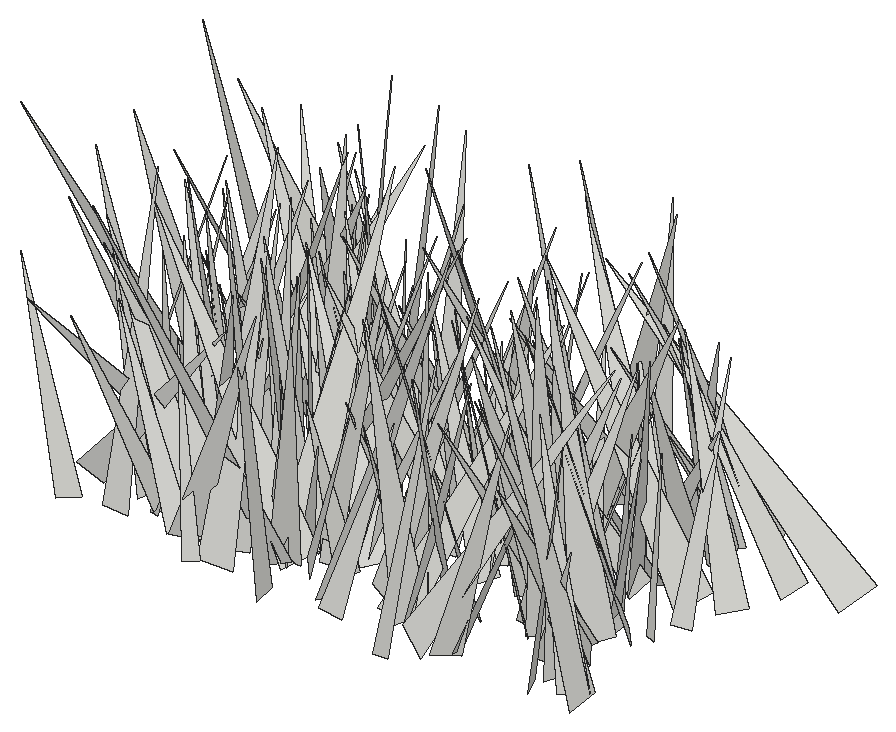
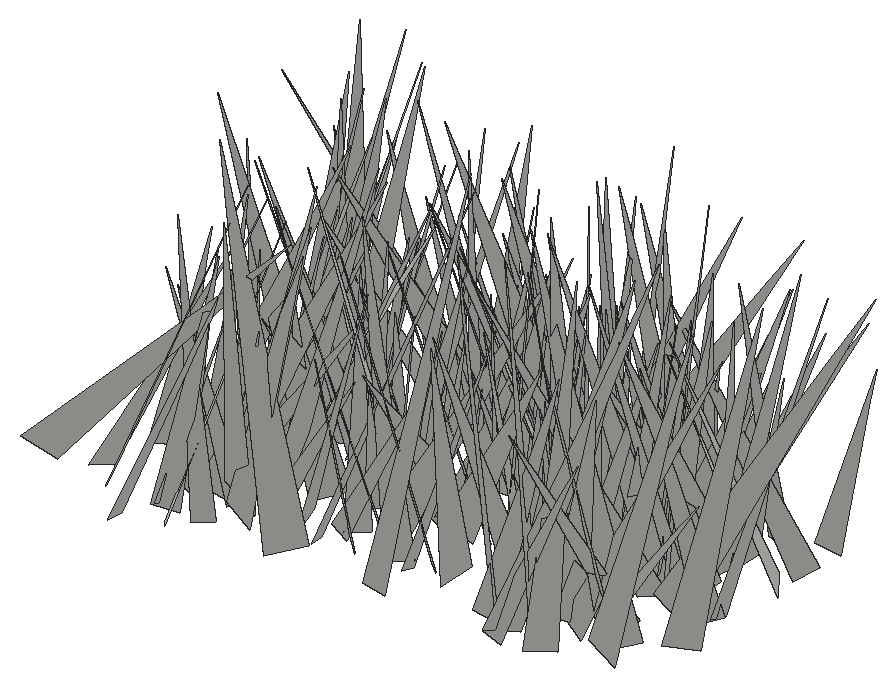
# SketchUp Ruby script. Lengths in inches.
U = 1.inch
M = Sketchup.active_model
def pt(a) = Geom::Point3d.new(a.map { |v| v * U })
def face(e, loops, mat)
  f = e.add_face(loops[0].map { |a| pt(a) })
  loops[1..].each { |l| e.add_face(l.map { |a| pt(a) }).erase! }
  f.material = f.back_material = mat if mat
  f
end
# faces: each face lists its corners as indices into pts; further lists are holes
def faces(e, pts, list, mat = nil) = list.each { |f| face(e, (f[0].is_a?(Array) ? f : [f]).map { |l| l.map { |i| pts[i] } }, mat) }
# xy, xz, yz: faces in a plane at the given z, y or x. An outline is a flat list of corners, or four numbers for a rectangle; further outlines are holes
def ring(l) = l.size == 4 ? [[l[0], l[1]], [l[2], l[1]], [l[2], l[3]], [l[0], l[3]]] : l.each_slice(2).to_a
def flat(e, list, mat, &to3) = list.each { |f| face(e, (f[0].is_a?(Array) ? f : [f]).map { |l| ring(l).map { |u, v| to3.(u, v) } }, mat) }
def xy(e, z, list, mat = nil) = flat(e, list, mat) { |x, y| [x, y, z] }
def xz(e, y, list, mat = nil) = flat(e, list, mat) { |x, z| [x, y, z] }
def yz(e, x, list, mat = nil) = flat(e, list, mat) { |y, z| [x, y, z] }
def lines(e, pts, list) = list.each { |a, b| e.add_line(pt(pts[a]), pt(pts[b])) }
# prism: a flat outline (further loops are holes) pulled along v
def prism(e, loops, v, mat = nil)
  f = face(e, loops, mat); d = Geom::Vector3d.new(v.map { |x| x * U })
  f.pushpull(f.normal.samedirection?(d) ? d.length : -d.length)
end
def box(e, o, s, mat = nil) = prism(e, [[o, [o[0] + s[0], o[1], o[2]], [o[0] + s[0], o[1] + s[1], o[2]], [o[0], o[1] + s[1], o[2]]]], [0, 0, s[2]], mat)
def at(x, y, z, deg = 0) = Geom::Transformation.translation(pt([x, y, z])) * Geom::Transformation.rotation(ORIGIN, Z_AXIS, deg.degrees)
def axes(o, x, y, z) = Geom::Transformation.new([*x, 0, *y, 0, *z, 0, *pt(o).to_a, 1])
def part(name) = M.definitions.add(name)
# library, detail: a bought-in or finely detailed component or shape, given as its bounding box
def library(name, o, s) = part(name).tap { |d| box(d.entities, o, s) }
def detail(e, o, s) = box(e.add_group.entities, o, s)
def put(e, d, t, mat = nil) = e.add_instance(d, t).tap { |i| i.material = mat if mat }
def group(e, t, mat = nil) = e.add_group.tap { |g| g.transformation = t; g.material = mat if mat }.entities
root = M.entities
c1 = part("fur_instance\#9")
p = [[0.8125,0,1.79],[0.67,-0.02,1.48],[0,-0.11,0],[0,0.11,0]]
faces(c1.entities,p,[[0,1,2,3]])
put(root,c1,axes([480.03,113.66,-21.86],[-7.83982,-0.95667,1.33619],[-0.96404,7.9519,0.03699],[1.33088,0.12461,7.89789]))
put(root,c1,axes([473.71,113.29,-21.86],[4.65487,-3.05281,1.35089],[-3.29302,-4.57961,0.99778],[-0.54826,1.58741,5.47649]))
put(root,c1,axes([465.41,112.65,-21.86],[-7.60319,-2.30719,2.08818],[-2.71089,7.61771,-1.45385],[1.52798,2.03457,7.8114]))
put(root,c1,axes([468.28,113.08,-21.86],[-0.49271,4.25835,1.65602],[4.30491,0.99075,-1.26683],[1.53091,-1.41548,4.0953]))
put(root,c1,axes([460.34,114.23,-21.86],[3.9818,-4.86666,0.84742],[-4.90357,-3.76221,1.43455],[0.59785,1.55519,6.12218]))
put(root,c1,axes([477.73,113.43,-21.86],[4.582,2.26461,1.64468],[2.3704,-4.81752,0.02956],[-1.48816,-0.70087,5.111]))
put(root,c1,axes([470.9,114.64,-21.86],[-5.74569,2.33772,2.68731],[2.89131,6.03979,0.92776],[2.08013,-1.9379,6.13328]))
put(root,c1,axes([464.3125,115.25,-21.86],[1.6892,-5.96403,1.00433],[-6.01842,-1.55459,0.89085],[0.59746,1.20222,6.13428]))
put(root,c1,axes([458.59,115.15,-21.66],[0.69444,-4.60057,1.02449],[-4.36557,-1.0182,-1.61314],[-1.77671,0.70364,4.36409]))
put(root,c1,axes([472.04,111.39,-21.66],[2.45384,5.3856,0.3895],[5.06414,-2.44383,1.88676],[-1.87372,0.44803,5.60947]))
put(root,c1,axes([478,116.68,-21.66],[-5.39374,-4.42373,0.73063],[-4.15874,5.36317,1.77113],[1.67573,-0.92879,6.74722]))
put(root,c1,axes([465.64,115.03,-21.66],[3.73133,2.74864,1.27928],[3.02044,-3.19509,-1.94493],[0.26177,-2.31318,4.20655]))
put(root,c1,axes([455.11,113.64,-21.66],[-1.60239,4.56784,1.22355],[4.62571,1.24567,1.40748],[-0.98238,-1.58525,4.63161]))
put(root,c1,axes([477.46,116.94,-21.86],[4.02503,-3.95124,0.17731],[-3.62061,-3.78264,-2.10414],[-1.59215,-1.38705,5.23314]))
put(root,c1,axes([469.98,115.76,-21.86],[-3.99319,-2.60087,1.40659],[-2.16034,4.18012,1.59628],[2.0189,-0.6713,4.49021]))
put(root,c1,axes([479.35,113.98,-21.86],[1.60632,-4.77246,2.92285],[-5.28453,-2.29441,-0.84211],[-1.84207,2.42054,4.96463]))
put(root,c1,axes([461.57,112.97,-21.86],[-0.27528,4.26527,0.41219],[4.05575,0.12601,1.40472],[-1.38323,-0.47937,4.03672]))
put(root,c1,axes([464.38,114.92,-21.86],[-3.051,-7.21191,1.32168],[-6.61753,2.09219,-3.8598],[-3.15701,2.58422,6.81338]))
put(root,c1,axes([471.67,116.11,-21.86],[-2.94569,-5.43055,1.36405],[-5.282,3.20651,1.35919],[1.85796,0.50597,6.02666]))
put(root,c1,axes([476.96,115.25,-21.86],[1.46313,-3.34357,0.17988],[-3.25058,-1.37123,0.95187],[0.80348,0.54115,3.52337]))
put(root,c1,axes([472.27,113.01,-21.66],[3.56611,7.00423,0.23479],[6.50816,-3.2121,-3.02618],[2.59966,-1.56674,7.25387]))
put(root,c1,axes([460,114.21,-21.66],[-2.19401,4.08598,0.64459],[3.98986,1.89782,1.55038],[-1.09165,-1.27572,4.37096]))
put(root,c1,axes([466.98,115.75,-21.86],[3.15907,-2.58161,1.45094],[-2.40771,-3.47422,-0.93937],[-1.72421,0.12146,3.97014]))
put(root,c1,axes([463.96,115.18,-21.86],[2.13967,5.72529,2.72362],[6.33838,-1.99885,-0.77766],[-0.14822,-2.82858,6.06237]))
put(root,c1,axes([464.82,115.5625,-21.86],[-6.95314,3.37085,0.59923],[3.40426,6.66259,2.02209],[-0.36434,-2.07731,7.45788]))
put(root,c1,axes([464.26,116.6875,-21.86],[-0.71595,-3.844,0.50308],[-3.36107,0.87042,1.86752],[1.93201,0.08975,3.4353]))
put(root,c1,axes([460.83,114.49,-21.86],[3.00603,-4.02582,3.59921],[-4.80148,-3.87769,-0.32715],[-2.47129,2.63706,5.01362]))
put(root,c1,axes([454.53,115.67,-21.66],[2.58062,-5.27777,0.62862],[-4.46822,-1.77579,3.43383],[2.87837,1.97518,4.76689]))
put(root,c1,axes([459.5,117.1,-21.66],[6.23542,-1.61716,0.46655],[-1.48447,-6.12774,-1.40019],[-0.79324,-1.24458,6.2877]))
put(root,c1,axes([475.46,117.84,-21.66],[5.45366,-4.66647,1.60556],[-4.21255,-5.64853,-2.10822],[-2.57063,-0.64365,6.86103]))
put(root,c1,axes([459.94,115.625,-21.66],[-5.34119,3.3335,0.99515],[3.47843,5.14626,1.43085],[0.05516,-1.74201,6.13133]))
put(root,c1,axes([469.27,115.0625,-21.66],[2.86437,6.58912,2.04567],[6.83224,-2.40073,-1.83379],[0.96006,-2.57407,6.94682]))
put(root,c1,axes([470.81,114.93,-21.86],[5.20805,0.62891,1.21236],[0.54515,-5.33937,0.42794],[-1.25226,0.29119,5.2284]))
put(root,c1,axes([457.89,119.08,-21.86],[3.04305,-5.48081,0.27728],[-4.42438,-2.6378,-3.58374],[-3.24669,-1.54241,5.14356]))
put(root,c1,axes([467.7,113.82,-21.66],[7.57177,-0.43303,1.80554],[-0.88332,-7.50835,1.90355],[-1.63317,2.05334,7.34137]))
put(root,c1,axes([472.63,116.49,-21.86],[-4.6315,-5.30606,1.24554],[-5.44783,4.55599,-0.84886],[0.16366,1.49838,6.99175]))
put(root,c1,axes([475.89,116.82,-21.86],[3.80262,-6.94068,2.14426],[-7.19034,-3.9408,-0.00453],[-1.0344,1.87826,7.9141]))
put(root,c1,axes([462.51,113.27,-21.86],[0.64716,8.27924,1.09317],[8.31403,-0.74193,0.69715],[-0.78591,-1.0312,8.27518]))
put(root,c1,axes([463.42,116.51,-21.86],[2.3019,2.88607,2.09295],[3.52279,-2.224,-0.8077],[-0.54756,-2.17555,3.60219]))
put(root,c1,axes([456.9,114.2,-21.86],[1.29784,6.7007,1.25957],[6.74597,-1.44798,0.75208],[-0.98888,-1.08363,6.78367]))
put(root,c1,axes([473.94,119.3125,-21.86],[-4.9139,-3.74374,0.55427],[-3.15126,4.55055,2.79845],[2.0958,-1.9355,5.50733]))
put(root,c1,axes([459.28,117.84,-21.66],[3.15853,-4.87453,2.05329],[-4.28659,-3.76007,-2.33247],[-3.09874,0.23284,5.31949]))
put(root,c1,axes([470.83,115.28,-21.86],[2.86323,5.98862,2.41998],[6.20716,-3.28322,0.78076],[-1.78634,-1.80966,6.59182]))
put(root,c1,axes([478.1,114.54,-21.86],[-7.47088,0.3057,1.86762],[-0.12287,7.51123,-1.721],[1.88848,1.69808,7.27638]))
put(root,c1,axes([474.64,117.06,-21.86],[0.98375,-3.96673,0.69714],[-3.91068,-0.76919,1.14174],[0.96305,0.9285,3.92417]))
put(root,c1,axes([469.9,115.8,-21.86],[-5.58164,-0.15602,0.84627],[-0.25003,5.60842,-0.61509],[0.82341,0.64537,5.54984]))
put(root,c1,axes([462.73,117.91,-21.86],[-2.8459,-6.01928,1.64103],[-5.98512,3.14324,1.14988],[1.76154,0.95508,6.5581]))
put(root,c1,axes([465.44,116.35,-21.86],[2.35807,6.09522,2.44102],[6.53945,-1.94795,-1.45322],[0.58808,-2.77931,6.37184]))
put(root,c1,axes([473.87,113.78,-21.86],[5.28462,2.45266,0.54887],[2.09175,-5.00051,2.20534],[-1.39334,1.79538,5.39252]))
put(root,c1,axes([457.11,115.91,-21.86],[-4.79431,0.50788,0.77321],[0.45097,4.84644,-0.38709],[0.80772,0.30866,4.80557]))
put(root,c1,axes([474.99,116.59,-21.86],[-4.95008,-4.07189,1.35786],[-4.2827,4.82407,-1.14641],[0.2873,1.75371,6.30629]))
put(root,c1,axes([457.57,116.89,-21.86],[1.09401,4.63876,2.44173],[5.21296,-1.22556,-0.00737],[-0.55243,-2.37843,4.76601]))
put(root,c1,axes([470.41,114.39,-21.86],[-2.47927,6.31853,1.78834],[5.49074,3.04318,-3.14001],[3.60191,-0.28983,6.01756]))
put(root,c1,axes([457.3,117.08,-21.86],[-7.08698,0.49693,1.41438],[0.58095,7.2106,0.37757],[1.38199,-0.48283,7.09434]))
put(root,c1,axes([476.7,117.58,-21.86],[-2.85824,2.70123,1.97363],[3.21945,2.92659,0.65696],[0.90938,-1.87078,3.87745]))
put(root,c1,axes([461.02,117.44,-21.86],[3.31439,2.62679,2.62231],[3.03004,-3.94532,0.12232],[-2.14367,-1.5153,4.22732]))
put(root,c1,axes([459.04,118.76,-21.66],[6.14406,2.36607,3.59044],[3.36505,-6.54408,-1.44586],[-2.67694,-2.79567,6.42319]))
put(root,c1,axes([467.88,118.56,-21.86],[-3.61169,-1.5954,0.61372],[-1.41522,3.59542,1.01805],[0.9587,-0.70282,3.81487]))
put(root,c1,axes([477.48,117.6,-21.86],[-6.5147,3.53544,2.59254],[3.94464,6.75335,0.70282],[1.91322,-1.88542,7.3788]))
put(root,c1,axes([463.09,117.92,-21.86],[1.22573,-5.85041,2.29876],[-6.17569,-1.55733,-0.67049],[-1.1715,2.08841,5.93971]))
put(root,c1,axes([475.56,118.7,-21.86],[3.66547,-5.8791,2.24711],[-5.89364,-4.11869,-1.16204],[-2.20868,1.23351,6.83002]))
put(root,c1,axes([463.05,118.49,-21.86],[5.57047,2.74276,2.66238],[3.42235,-5.67452,-1.31471],[-1.7025,-2.43273,6.06831]))
put(root,c1,axes([466.36,117.43,-21.86],[4.41432,4.17138,0.78555],[4.1779,-4.06951,-1.86761],[0.75011,-1.88212,5.77916]))
put(root,c1,axes([462.77,114.4,-21.66],[1.87355,6.48838,0.26131],[6.01197,-1.83596,2.48253],[-2.45429,0.45575,6.28063]))
put(root,c1,axes([459.07,115.54,-21.86],[-1.28039,5.01222,0.36244],[4.5705,1.31696,-2.06622],[2.08908,0.19072,4.74262]))
put(root,c1,axes([476.73,120.1,-21.86],[-3.9391,-6.11846,0.96009],[-6.01065,4.05101,1.1555],[1.49311,0.1661,7.18449]))
put(root,c1,axes([455.02,120.4,-21.66],[-6.16239,-2.08969,1.53365],[-1.42213,6.03269,2.50561],[2.16712,-1.98337,6.00531]))
put(root,c1,axes([473.29,118.72,-21.86],[0.8668,-4.44855,1.11397],[-4.54098,-0.99091,-0.42373],[-0.6404,1.00517,4.51236]))
put(root,c1,axes([478.28,118.76,-21.86],[-5.08924,-4.37631,0.84531],[-4.44671,5.07308,-0.50754],[0.30556,0.93743,6.69289]))
put(root,c1,axes([458.24,114.92,-21.86],[3.80784,5.11048,0.67094],[4.57882,-3.73693,2.47721],[-2.36675,0.99257,5.87197]))
put(root,c1,axes([459.27,118.14,-21.86],[1.7878,3.1828,1.34143],[3.44443,-1.53093,-0.95817],[0.2561,-1.62848,3.52255]))
put(root,c1,axes([465.95,116,-21.86],[1.51119,6.34193,0.92742],[6.21067,-1.68435,1.39797],[-1.58356,-0.55387,6.36784]))
put(root,c1,axes([464.27,116.01,-21.66],[-3.17908,7.18759,1.82609],[7.05927,3.54175,-1.65087],[2.27218,-0.9472,7.68392]))
put(root,c1,axes([462.32,117.93,-21.86],[5.04239,2.3615,1.06864],[2.46365,-5.09289,-0.37039],[-0.80566,-0.79378,5.55564]))
put(root,c1,axes([467.25,117.21,-21.86],[-4.13597,4.87198,0.25098],[4.78591,3.98836,1.44689],[-0.94567,-1.12348,6.22487]))
put(root,c1,axes([475.26,117.24,-21.66],[0.44188,5.84269,1.52194],[5.83939,-0.02571,-1.59672],[1.53457,-1.58458,5.63763]))
put(root,c1,axes([459.37,117.79,-21.86],[-1.25475,3.57203,1.31412],[3.70812,1.4592,-0.42579],[0.858,-1.08261,3.76198]))
put(root,c1,axes([472.83,119.73,-21.86],[-3.85431,-2.63258,1.04926],[-2.43046,3.98156,1.06172],[1.4575,-0.32233,4.54521]))
put(root,c1,axes([463.2,116.15,-21.66],[1.09357,6.43106,0.77169],[6.11568,-1.28298,2.02542],[-2.13365,-0.38127,6.20097]))
put(root,c1,axes([459.51,118.24,-21.86],[4.90342,0.51596,3.18153],[0.4361,-5.84514,0.27581],[-3.19346,-0.00597,4.92277]))
put(root,c1,axes([477.33,118.9,-21.86],[4.21688,0.53755,0.91963],[0.65776,-4.26755,-0.52159],[-0.83787,-0.64478,4.21888]))
put(root,c1,axes([459.23,118.26,-21.86],[-2.59565,5.50063,1.7013],[5.74289,2.3395,1.19781],[-0.41302,-2.03926,5.96319]))
put(root,c1,axes([461.44,119.17,-21.86],[-3.39336,2.50243,2.08506],[2.97495,3.60715,0.51243],[1.32637,-1.68843,4.18502]))
put(root,c1,axes([462.08,119.02,-21.86],[-2.18081,-4.36379,1.96245],[-4.63729,2.45895,0.31456],[1.17875,1.60022,4.86823]))
put(root,c1,axes([463.74,117.52,-21.66],[7.28902,-0.71217,0.57332],[-0.83779,-7.04721,1.89755],[-0.36604,1.94818,7.07364]))
put(root,c1,axes([456.89,121.07,-21.66],[-1.39061,-8.04384,0.83594],[-7.45661,0.94696,-3.29214],[-3.13068,1.31752,7.46987]))
put(root,c1,axes([457.53,120.53,-21.66],[-3.39488,-3.98848,1.56761],[-3.7052,3.73666,1.48306],[2.15333,0.14147,5.02331]))
put(root,c1,axes([477.62,118.89,-21.86],[-4.70558,-0.80345,0.83315],[-0.88013,4.74917,-0.39105],[0.7517,0.53106,4.75763]))
put(root,c1,axes([476.7,117.73,-21.66],[-6.97142,-3.26118,0.0354],[-2.96258,6.29742,-3.28677],[-1.3637,2.99072,6.9594]))
put(root,c1,axes([468.02,120.58,-21.66],[-6.07615,0.58264,0.90457],[0.83184,5.83413,1.82981],[0.68247,-1.92372,5.8233]))
put(root,c1,axes([467.43,117.99,-21.66],[-3.01404,5.97197,0.86388],[5.95256,2.78442,1.51964],[-0.98886,-1.44144,6.51457]))
put(root,c1,axes([456.87,118.66,-21.86],[6.22243,-0.20354,0.93497],[-0.30289,-6.25415,0.65425],[-0.90767,0.69164,6.19128]))
put(root,c1,axes([454.84,116.98,-21.66],[5.18703,3.91751,0.7095],[3.72248,-5.18551,1.41748],[-1.41191,0.72053,6.34373]))
put(root,c1,axes([471.28,118.72,-21.86],[-5.48361,2.04542,0.49712],[2.0602,5.49974,0.09665],[0.43181,-0.2646,5.85187]))
put(root,c1,axes([474.8,120.47,-21.86],[-6.27523,-0.24227,0.55286],[-0.1392,6.19931,1.13667],[0.58735,-1.11924,6.17618]))
put(root,c1,axes([471.85,120.27,-21.86],[-0.67343,-4.75938,1.30258],[-4.88536,0.82798,0.49956],[0.69398,1.21023,4.78075]))
put(root,c1,axes([477,119.62,-21.86],[4.07501,0.67414,1.38281],[0.80205,-4.27202,-0.28088],[-1.31276,-0.5174,4.12083]))
put(root,c1,axes([460.21,119.67,-21.86],[-6.22894,0.57755,1.75246],[0.68588,6.45268,0.31131],[1.71297,-0.48351,6.24791]))
put(root,c1,axes([463.89,118.26,-21.86],[4.96936,4.425,0.65774],[4.44372,-4.99597,0.03757],[-0.51632,-0.4092,6.65385]))
put(root,c1,axes([476.49,121.625,-21.66],[-4.86866,0.51762,1.11395],[0.97098,4.41082,2.19421],[0.75234,-2.34296,4.3769]))
put(root,c1,axes([464.43,118.32,-21.86],[-5.98582,-0.44068,0.88109],[-0.67667,5.78235,-1.70504],[0.71598,1.78068,5.75475]))
put(root,c1,axes([472.82,119.57,-21.66],[2.29321,-4.71361,1.70331],[-4.8602,-1.63403,2.02152],[1.22385,2.34308,4.83635]))
put(root,c1,axes([457.65,117.08,-21.66],[-5.19171,3.73852,1.55221],[3.028,5.26206,-2.54592],[2.68647,1.29382,5.8693]))
put(root,c1,axes([463.51,118.41,-21.86],[3.13584,4.70476,0.63652],[4.72939,-3.16238,0.0748],[-0.41563,-0.48786,5.65355]))
put(root,c1,axes([478.97,119.13,-21.86],[1.67627,3.15128,1.04901],[3.10636,-1.90337,0.75402],[-1.17538,-0.53615,3.48882]))
put(root,c1,axes([457.81,119.16,-21.86],[2.77668,6.00015,1.42785],[6.14966,-2.57364,-1.14395],[0.47149,-1.76779,6.51177]))
put(root,c1,axes([475.85,117.9,-21.86],[3.6245,2.89722,0.22495],[2.66528,-3.45765,1.58821],[-1.15791,1.11007,4.35987]))
put(root,c1,axes([458.65,119.17,-21.86],[7.58645,0.4489,1.20084],[0.2907,-7.62155,1.01257],[-1.24861,0.95304,7.53196]))
put(root,c1,axes([455.08,120.75,-21.66],[2.87453,-4.20489,0.68169],[-4.14129,-2.56592,1.63539],[0.99777,1.46412,4.82385]))
put(root,c1,axes([463.42,119.92,-21.86],[-4.19942,1.95994,0.17006],[1.96728,4.18576,0.33862],[0.01038,-0.37878,4.62189]))
put(root,c1,axes([476.16,121.75,-21.66],[6.10646,0.88523,1.50787],[1.27518,-6.00248,-1.64024],[-1.19633,-1.87958,5.94829]))
put(root,c1,axes([462.28,121.07,-21.86],[-1.89592,-3.45095,1.30694],[-3.60556,2.04518,0.16982],[0.78554,1.05823,3.9338]))
put(root,c1,axes([470.73,119.98,-21.86],[-1.71851,4.03919,1.0736],[4.16688,1.74577,0.10182],[0.32374,-1.02868,4.3884]))
put(root,c1,axes([472.63,121.92,-21.86],[3.82613,-7.13137,0.63835],[-6.75778,-3.35774,2.99351],[2.36564,1.94225,7.51895]))
put(root,c1,axes([462.73,122.26,-21.86],[1.15457,-5.41906,0.82486],[-5.48032,-1.12384,0.28761],[0.11275,0.86626,5.53322]))
put(root,c1,axes([462.1,120.15,-21.86],[-4.21577,-3.58718,3.5566],[-4.31781,4.96325,-0.11214],[2.62178,2.40587,5.53425]))
put(root,c1,axes([459.37,124.17,-21.66],[4.70734,-3.12135,0.14145],[-2.64852,-4.12178,-2.81392],[-1.65776,-2.27815,4.89732]))
put(root,c1,axes([469.6875,120.97,-21.86],[-3.40834,-0.81843,0.94444],[-0.85751,3.5273,-0.03792],[0.90911,0.25869,3.50503]))
put(root,c1,axes([467.59,120.24,-21.86],[-3.65849,-0.26653,0.63033],[-0.40108,3.61269,-0.80033],[0.55452,0.85461,3.57982]))
put(root,c1,axes([470.83,119.07,-21.86],[1.97963,5.14738,0.61551],[5.06452,-2.06097,0.94673],[-1.10678,-0.22402,5.43306]))
put(root,c1,axes([478.77,122.02,-21.66],[-7.28796,2.50197,0.93453],[2.66483,6.99355,2.0583],[0.17855,-2.25345,7.42547]))
put(root,c1,axes([469.22,122.36,-21.86],[-0.65869,-6.64833,1.3688],[-6.16249,0.00919,-2.92087],[-2.84565,1.51902,6.00855]))
put(root,c1,axes([469.34,121.96,-21.86],[4.68379,1.41709,0.13919],[1.37897,-4.39495,-1.65779],[0.35492,-1.62533,4.60411]))
put(root,c1,axes([468.23,121.02,-21.86],[-1.43157,-3.77915,1.63266],[-4.11341,1.2436,-0.72817],[-0.16553,1.78,3.97506]))
put(root,c1,axes([476.31,118.8,-21.86],[0.39127,5.5531,0.09038],[5.24022,-0.39914,1.8382],[-1.83989,0.04412,5.25462]))
put(root,c1,axes([461.53,121.08,-21.86],[6.01123,-4.10409,2.83515],[-4.50522,-6.3728,0.32708],[-2.14119,1.8869,7.27128]))
put(root,c1,axes([474.37,122.83,-21.86],[-6.75805,0.02177,1.99006],[0.56326,6.77748,1.83863],[1.90881,-1.92284,6.50317]))
put(root,c1,axes([463.1875,121.03,-21.86],[4.07736,0.20577,0.16386],[0.20057,-4.0788,0.13116],[-0.17019,0.12285,4.08044]))
put(root,c1,axes([469.91,121.42,-21.86],[-3.21218,-2.63282,1.4726],[-2.81239,3.39173,-0.07071],[1.09119,0.99138,4.15269]))
put(root,c1,axes([469.33,121.28,-21.86],[6.01088,3.96881,0.98389],[4.08835,-5.80352,-1.56674],[0.06989,-1.84874,7.03046]))
put(root,c1,axes([469.83,120.625,-21.86],[1.94279,3.86541,2.10519],[3.74501,-2.66073,1.42935],[-2.3126,-1.06149,4.08323]))
put(root,c1,axes([465.61,121.12,-21.66],[4.35224,4.23695,0.82253],[4.28263,-4.09432,-1.57033],[0.53605,-1.68972,5.86752]))
put(root,c1,axes([454.67,123.08,-21.66],[4.91943,-4.73173,2.30235],[-4.40019,-5.42749,-1.75256],[-2.8859,0.2095,6.59686]))
put(root,c1,axes([462.71,119.88,-21.86],[-2.92778,3.00983,0.00711],[2.98882,2.90849,-0.48849],[0.35507,0.33555,4.17041]))
put(root,c1,axes([462.8,121.13,-21.86],[-6.11884,4.72961,1.11538],[4.85918,5.97068,1.339],[0.0418,-1.7422,7.61686]))
put(root,c1,axes([464.04,122.14,-21.86],[-6.4664,-4.252,2.80304],[-4.40658,6.94256,0.3657],[2.55316,1.21333,7.73047]))
put(root,c1,axes([476.04,124.77,-21.66],[2.18391,-6.70079,0.42323],[-6.08063,-2.16263,-2.86325],[-2.84706,-0.52116,6.43986]))
put(root,c1,axes([462.375,122.73,-21.86],[-1.26664,-5.03308,1.07763],[-5.14261,1.28411,-0.04714],[0.2163,1.05675,5.1898]))
put(root,c1,axes([476.62,122.62,-21.86],[-2.08934,-4.39389,0.06996],[-3.98317,1.86084,-2.08523],[-1.85622,0.95264,4.39584]))
put(root,c1,axes([470.11,123.42,-21.86],[4.2644,-2.86076,0.08373],[-2.8192,-4.22473,-0.76148],[-0.49304,-0.58632,5.07831]))
put(root,c1,axes([464.625,121.78,-21.86],[-3.23296,-4.09809,2.47034],[-4.47809,3.64184,0.18098],[1.68632,1.81429,5.21667]))
put(root,c1,axes([470.7,125.18,-21.66],[-6.78403,-3.28205,0.63683],[-2.89291,6.48484,2.60352],[1.67585,-2.09175,7.07224]))
put(root,c1,axes([456.71,124.15,-21.86],[3.10816,-7.62871,0.22312],[-7.12075,-2.81203,3.04879],[2.74626,1.34273,7.65263]))
put(root,c1,axes([462,123.125,-21.86],[5.00049,1.26706,0.71261],[1.41038,-4.84715,-1.27832],[-0.35226,-1.4205,4.99762]))
put(root,c1,axes([476.59,124.64,-21.86],[5.34642,-2.10558,1.0321],[-1.67954,-5.23165,-1.97278],[-1.63641,-1.50973,5.39684]))
put(root,c1,axes([468.89,119.21,-21.66],[-4.90566,2.32822,0.51514],[1.6552,4.17303,-3.098],[1.71648,2.62995,4.45965]))
put(root,c1,axes([466.82,124.52,-21.86],[-4.80536,-1.45342,1.08645],[-0.98448,4.67157,1.89512],[1.52434,-1.5647,4.64891]))
put(root,c1,axes([459.08,124.1875,-21.86],[-2.83632,-6.0499,0.28173],[-5.90232,2.69141,-1.62612],[-1.35766,0.93829,6.48088]))
put(root,c1,axes([458,120.61,-21.66],[0.84349,7.5995,0.98427],[7.14395,-0.42161,-2.86687],[2.77222,-1.22577,7.08837]))
put(root,c1,axes([469.55,122.74,-21.86],[5.84897,4.9177,0.90335],[4.92852,-5.43629,-2.31659],[0.84231,-2.33947,7.282]))
put(root,c1,axes([479.375,120.53,-21.86],[0.66443,5.27954,0.01832],[5.19176,-0.65673,0.9642],[-0.95891,0.10252,5.2331]))
put(root,c1,axes([467.48,124.18,-21.86],[0.87943,-6.58228,1.27772],[-6.45662,-0.48373,1.95201],[1.80858,1.47376,6.34739]))
put(root,c1,axes([458.42,123,-21.86],[-2.80536,-2.90649,0.0794],[-2.63209,2.49174,-1.78533],[-1.23535,1.29136,3.62358]))
put(root,c1,axes([470.7,121.62,-21.86],[-2.98771,2.56269,0.00271],[2.54357,2.96592,-0.47684],[0.31249,0.36018,3.90722]))
put(root,c1,axes([480.09,122.7,-21.86],[-4.17135,3.80631,1.04328],[3.93898,4.10999,0.75433],[0.24669,-1.26356,5.59635]))
put(root,c1,axes([466.95,121.41,-21.66],[-1.95645,6.57203,0.15793],[5.85701,1.66776,3.15567],[-2.98529,-1.03499,6.08778]))
put(root,c1,axes([461.98,121.9,-21.86],[0.78619,5.10987,0.99795],[4.99569,-1.02461,1.31074],[-1.46621,-0.75112,5.00108]))
put(root,c1,axes([473.91,123.375,-21.86],[-2.56697,2.61634,0.35758],[2.51502,2.27032,1.44317],[-0.80484,-1.25014,3.36925]))
put(root,c1,axes([474.21,124.86,-21.86],[-2.28168,-4.43341,1.38047],[-4.1851,2.6298,1.52839],[2.0114,0.44265,4.74608]))
put(root,c1,axes([466.64,126.79,-21.66],[-3.41876,-7.6362,0.72671],[-7.48826,3.49493,1.49637],[1.66304,0.03883,8.23167]))
put(root,c1,axes([470.64,123.89,-21.86],[-1.09532,-3.977,1.33167],[-3.82769,0.38536,-1.99748],[-1.71426,1.68065,3.6092]))
put(root,c1,axes([460.96,122.57,-21.86],[-4.7564,-0.43454,1.78324],[-0.95829,4.81251,-1.3833],[1.56539,1.62573,4.5715]))
put(root,c1,axes([463.23,122.33,-21.86],[5.70541,0.17051,1.69377],[-0.31532,-5.71566,1.63753],[-1.67287,1.65887,5.46803]))
put(root,c1,axes([474.83,124.87,-21.66],[1.43751,-4.12245,0.23292],[-3.7226,-1.18725,1.96162],[1.78636,0.84328,3.90039]))
put(root,c1,axes([460.84,126.28,-21.66],[-7.92224,1.63819,2.17065],[2.33717,7.51957,2.85498],[1.39032,-3.306,7.56932]))
put(root,c1,axes([458.68,126.625,-21.66],[6.56004,-2.8558,0.90961],[-2.50702,-6.42798,-2.10074],[-1.6425,-1.59457,6.83935]))
put(root,c1,axes([465.9,124.08,-21.66],[4.67492,4.49227,1.13099],[4.6277,-4.45606,-1.42912],[0.20972,-1.8104,6.324]))
put(root,c1,axes([477.51,124.81,-21.86],[-2.10468,-4.52268,1.53831],[-4.75533,2.14388,-0.20306],[0.45584,1.48319,4.98428]))
put(root,c1,axes([476.22,127.53,-21.86],[-4.88167,-3.98465,0.29136],[-3.56929,4.55624,2.50876],[1.79514,-1.77658,5.7805]))
put(root,c1,axes([457.39,123.82,-21.86],[3.97347,4.57155,1.31094],[4.73936,-3.94824,-0.59665],[-0.39506,-1.38509,6.02757]))
put(root,c1,axes([475.7,123.68,-21.86],[-6.02819,4.2729,0.70004],[4.32885,5.97346,0.81585],[0.09372,-1.07093,7.34378]))
put(root,c1,axes([460.55,122.4375,-21.66],[-2.20757,6.36235,0.08993],[6.1827,2.12231,1.62203],[-1.50393,-0.61421,6.5362]))
put(root,c1,axes([475.82,123.68,-21.86],[-3.58743,2.64736,0.43412],[2.66538,3.59954,0.07504],[0.30449,-0.3184,4.45786]))
put(root,c1,axes([480.94,125.41,-21.86],[-5.72955,1.74546,0.28048],[1.75274,5.48455,1.67353],[-0.23061,-1.68113,5.75097]))
put(root,c1,axes([477.19,126.73,-21.66],[-3.37323,-1.69913,0.74168],[-1.13548,3.11072,1.96213],[1.46554,-1.50074,3.22735]))
put(root,c1,axes([457.84,122.43,-21.86],[-0.63862,5.35473,0.03552],[5.1577,0.62471,-1.44573],[1.43964,0.13724,5.19527]))
put(root,c1,axes([480.17,125.85,-21.86],[-6.75441,-2.93713,0.31923],[-2.94167,6.75982,-0.04619],[0.27431,0.1697,7.36523]))
put(root,c1,axes([456.77,125.3,-21.66],[-2.69995,-7.06667,2.40673],[-7.39529,2.18224,-1.88876],[-1.01973,2.88442,7.32531]))
put(root,c1,axes([474.43,125.29,-21.86],[1.71463,6.79892,3.94816],[7.36353,-2.80488,1.63226],[-2.7553,-3.26505,6.81916]))
put(root,c1,axes([474.93,126.77,-21.66],[0.27487,-5.90315,0.86813],[-5.62576,0.03312,2.00651],[1.98787,0.91,5.55848]))
put(root,c1,axes([471.32,126.26,-21.86],[6.86151,-4.43995,0.81428],[-4.49635,-6.85344,0.51929],[-0.39875,0.87961,8.15621]))
put(root,c1,axes([483.4,126.17,-21.66],[-5.86481,5.71927,0.12396],[4.62698,4.63811,4.91939],[-3.36399,-3.59156,6.55024]))
put(root,c1,axes([472.15,124.05,-21.86],[-7.13799,-1.18277,0.6594],[-1.323,6.84565,-2.04241],[0.28881,2.12669,6.94107]))
put(root,c1,axes([476.96,126.56,-21.86],[1.57492,-4.967,1.49516],[-5.0252,-1.8484,-0.84719],[-1.28605,1.13987,5.14138]))
put(root,c1,axes([459.56,125.8125,-21.86],[6.90611,3.10223,2.59996],[3.46907,-7.18559,-0.64093],[-2.08547,-1.6797,7.5437]))
put(root,c1,axes([469.66,124.3125,-21.86],[2.96652,3.66752,1.13191],[3.55325,-3.16507,0.94281],[-1.45132,-0.25254,4.62191]))
put(root,c1,axes([478.05,128.26,-21.86],[-6.75502,-2.37628,0.59319],[-2.11002,6.52988,2.13012],[1.24354,-1.82836,6.83664]))
put(root,c1,axes([461.35,125.98,-21.86],[-4.14785,-5.45032,3.6874],[-5.74845,5.12259,1.10541],[3.20285,2.13555,6.75935]))
put(root,c1,axes([461.88,125.83,-21.66],[-1.46223,5.38545,2.28823],[5.73287,0.84616,1.67196],[-1.17188,-2.58033,5.32407]))
put(root,c1,axes([461.02,126.66,-21.86],[-0.44719,-4.16584,0.88919],[-4.01944,0.11666,-1.47491],[-1.41032,0.98845,3.92158]))
put(root,c1,axes([474.875,124.6875,-21.86],[0.75585,6.87514,1.87347],[7.05211,-0.99202,0.79528],[-1.02238,-1.75986,6.87069]))
put(root,c1,axes([465.03,123.8,-21.86],[-6.34351,2.24327,1.15963],[1.89857,6.30395,-1.80908],[1.66506,1.35834,6.48071]))
